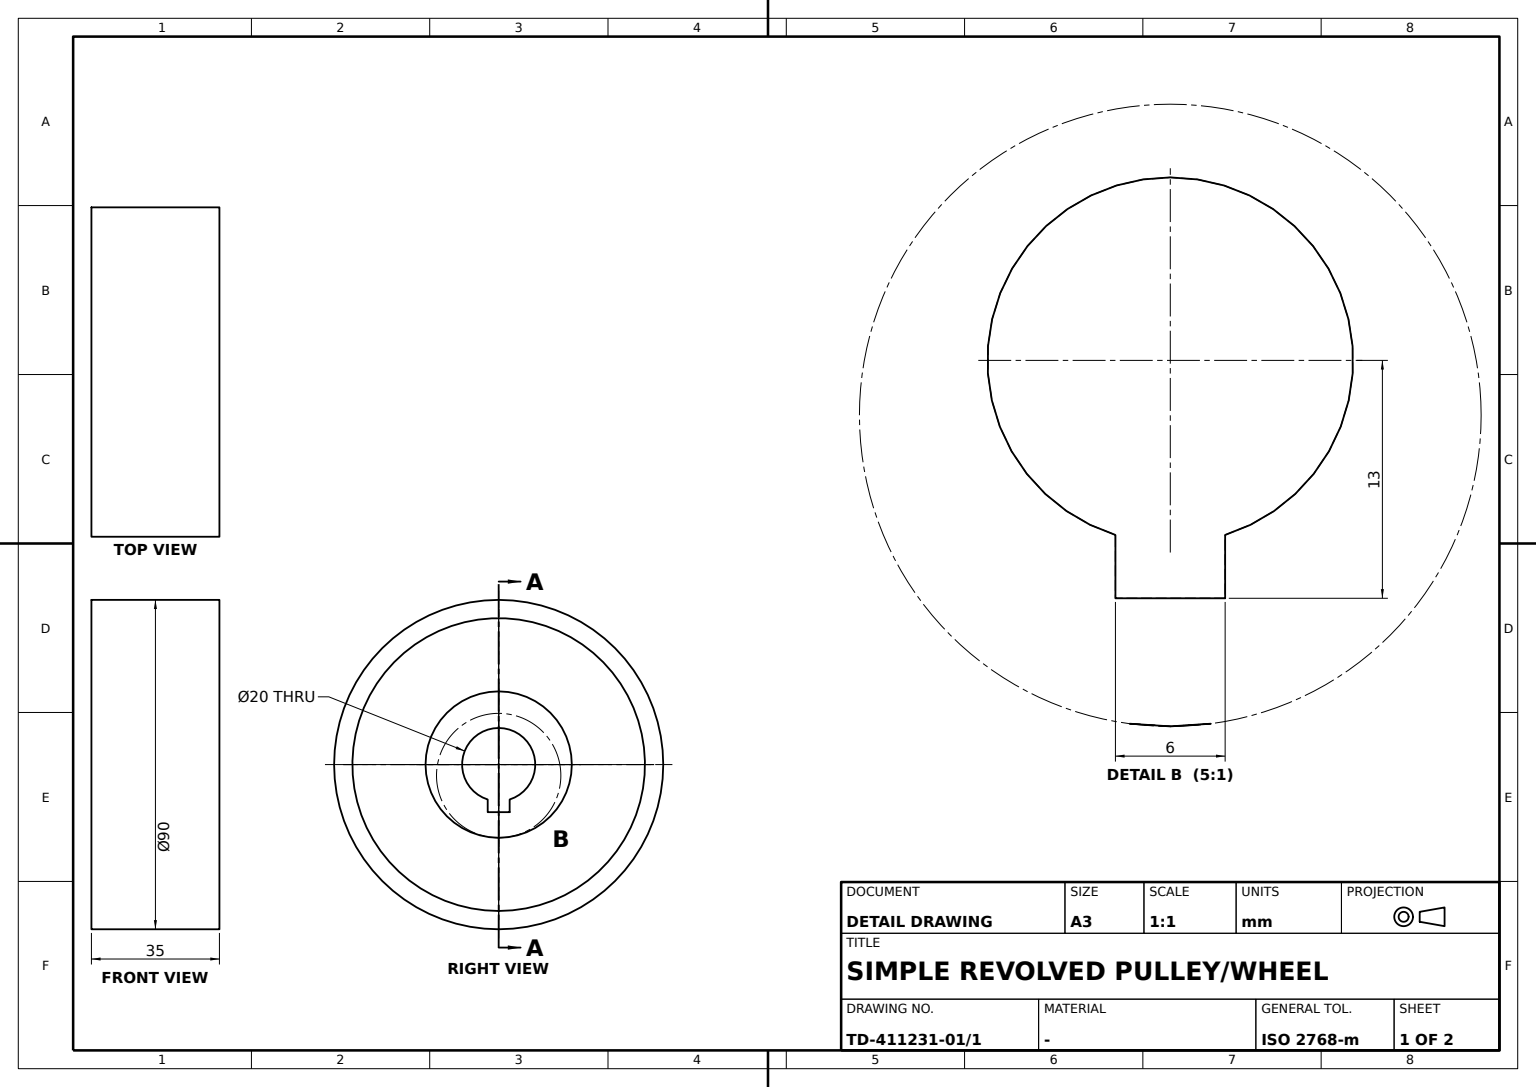
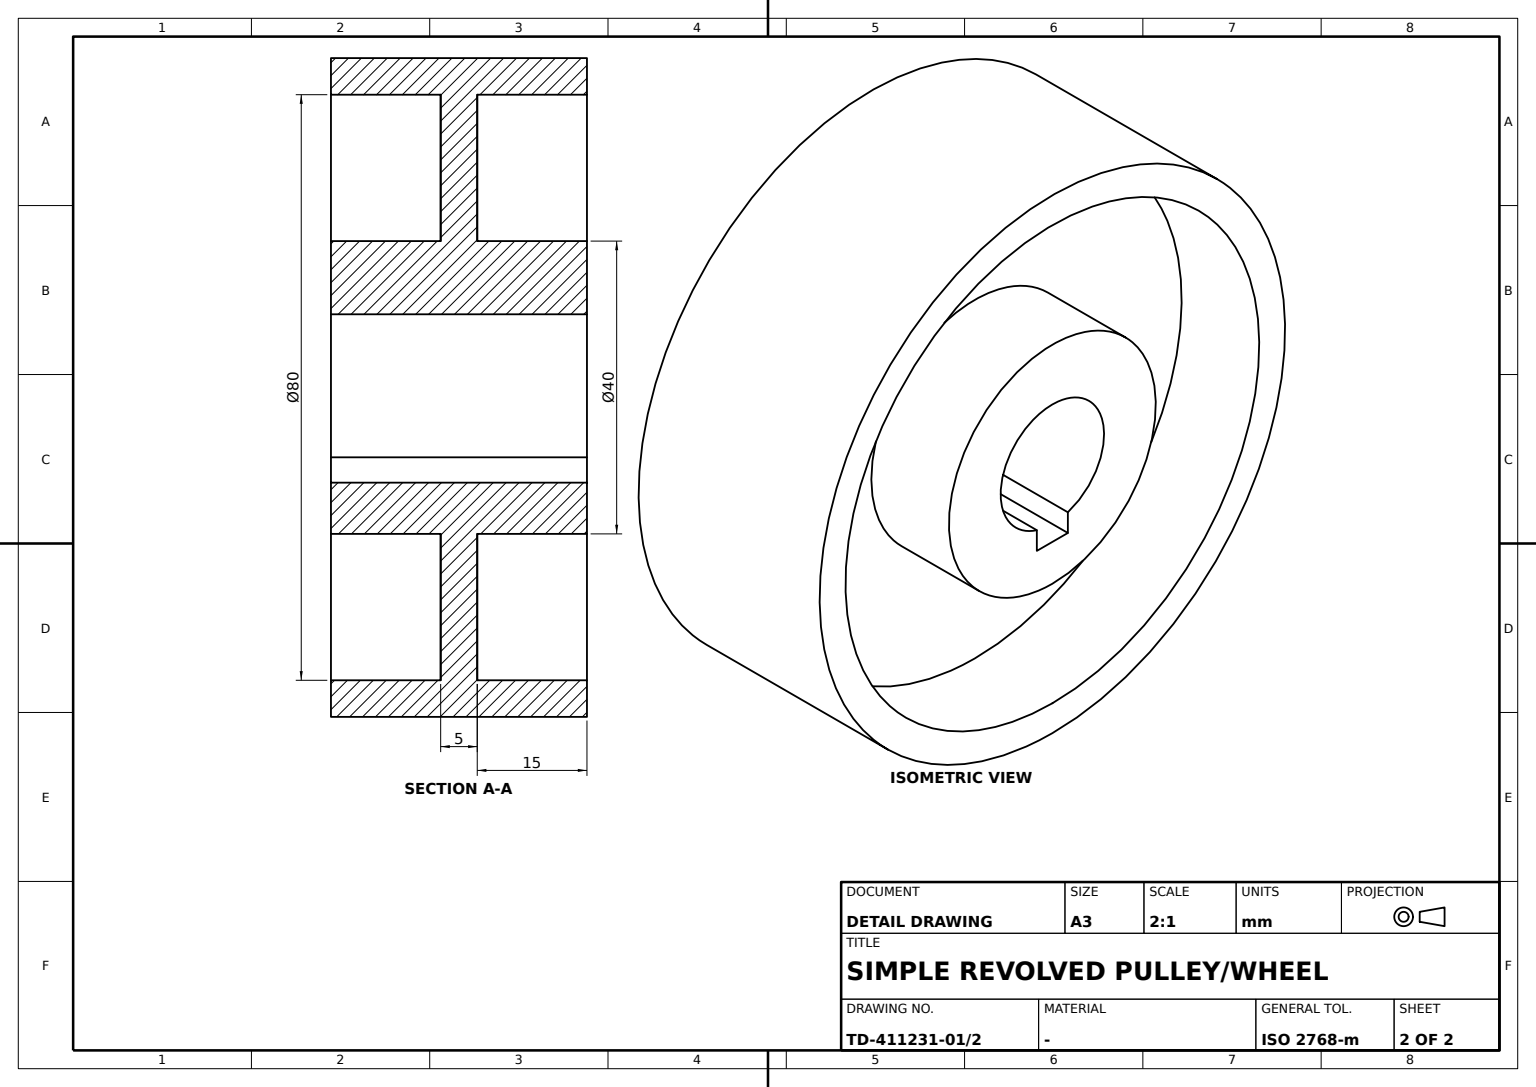
ISO-10303-21;
HEADER;
FILE_DESCRIPTION((''),'2;1');
FILE_NAME('','',(''),(''),'','','');
FILE_SCHEMA(('AUTOMOTIVE_DESIGN'));
ENDSEC;
DATA;
#1=APPLICATION_CONTEXT('');
#2=PRODUCT_CONTEXT('',#1,'mechanical');
#3=PRODUCT('','','',(#2));
#4=PRODUCT_DEFINITION_FORMATION('','',#3);
#5=PRODUCT_DEFINITION_CONTEXT('',#1,'design');
#6=PRODUCT_DEFINITION('','',#4,#5);
#7=PRODUCT_DEFINITION_SHAPE('','',#6);
#8=(LENGTH_UNIT()NAMED_UNIT(*)SI_UNIT(.MILLI.,.METRE.));
#9=(NAMED_UNIT(*)PLANE_ANGLE_UNIT()SI_UNIT($,.RADIAN.));
#10=(NAMED_UNIT(*)SI_UNIT($,.STERADIAN.)SOLID_ANGLE_UNIT());
#11=UNCERTAINTY_MEASURE_WITH_UNIT(LENGTH_MEASURE(0.005),#8,'distance_accuracy_value','');
#12=(GEOMETRIC_REPRESENTATION_CONTEXT(3)GLOBAL_UNCERTAINTY_ASSIGNED_CONTEXT((#11))GLOBAL_UNIT_ASSIGNED_CONTEXT((#8,#9,#10))REPRESENTATION_CONTEXT('',''));
#13=CARTESIAN_POINT('',(17.5,-3.,-13.));
#14=VERTEX_POINT('',#13);
#15=CARTESIAN_POINT('',(-17.5,-3.,-13.));
#16=VERTEX_POINT('',#15);
#17=DIRECTION('',(-1.,0.,0.));
#18=VECTOR('',#17,1000.);
#19=LINE('',#13,#18);
#20=EDGE_CURVE('',#14,#16,#19,.T.);
#21=ORIENTED_EDGE('',*,*,#20,.T.);
#22=CARTESIAN_POINT('',(-17.5,-3.,-9.539392));
#23=VERTEX_POINT('',#22);
#24=CARTESIAN_POINT('',(-17.5,-3.,-6.63467));
#25=DIRECTION('',(0.,0.,-1.));
#26=VECTOR('',#25,1000.);
#27=LINE('',#24,#26);
#28=EDGE_CURVE('',#23,#16,#27,.T.);
#29=ORIENTED_EDGE('',*,*,#28,.F.);
#30=CARTESIAN_POINT('',(17.5,-3.,-9.539392));
#31=VERTEX_POINT('',#30);
#32=DIRECTION('',(1.,0.,0.));
#33=VECTOR('',#32,1000.);
#34=LINE('',#22,#33);
#35=EDGE_CURVE('',#23,#31,#34,.T.);
#36=ORIENTED_EDGE('',*,*,#35,.T.);
#37=CARTESIAN_POINT('',(17.5,-3.,-6.63467));
#38=LINE('',#37,#26);
#39=EDGE_CURVE('',#31,#14,#38,.T.);
#40=ORIENTED_EDGE('',*,*,#39,.T.);
#41=EDGE_LOOP('',(#21,#29,#36,#40));
#42=FACE_BOUND('',#41,.T.);
#43=DIRECTION('',(0.,1.,0.));
#44=AXIS2_PLACEMENT_3D('',#37,#43,#25);
#45=PLANE('',#44);
#46=ADVANCED_FACE('',(#42),#45,.T.);
#47=CARTESIAN_POINT('',(17.5,0.,-45.));
#48=VERTEX_POINT('',#47);
#49=CARTESIAN_POINT('',(17.5,0.,0.));
#50=AXIS2_PLACEMENT_3D('',#49,#32,#25);
#51=CIRCLE('',#50,45.);
#52=EDGE_CURVE('',#48,#48,#51,.T.);
#53=ORIENTED_EDGE('',*,*,#52,.T.);
#54=EDGE_LOOP('',(#53));
#55=FACE_BOUND('',#54,.T.);
#56=CARTESIAN_POINT('',(17.5,0.,-40.));
#57=VERTEX_POINT('',#56);
#58=CIRCLE('',#50,40.);
#59=EDGE_CURVE('',#57,#57,#58,.T.);
#60=ORIENTED_EDGE('',*,*,#59,.F.);
#61=EDGE_LOOP('',(#60));
#62=FACE_BOUND('',#61,.T.);
#63=CARTESIAN_POINT('',(17.5,20.,0.));
#64=AXIS2_PLACEMENT_3D('',#63,#32,#43);
#65=PLANE('',#64);
#66=ADVANCED_FACE('',(#55,#62),#65,.T.);
#67=ORIENTED_EDGE('',*,*,#52,.F.);
#68=EDGE_LOOP('',(#67));
#69=FACE_BOUND('',#68,.T.);
#70=CARTESIAN_POINT('',(-17.5,0.,-45.));
#71=VERTEX_POINT('',#70);
#72=CARTESIAN_POINT('',(-17.5,0.,0.));
#73=AXIS2_PLACEMENT_3D('',#72,#32,#25);
#74=CIRCLE('',#73,45.);
#75=EDGE_CURVE('',#71,#71,#74,.T.);
#76=ORIENTED_EDGE('',*,*,#75,.T.);
#77=EDGE_LOOP('',(#76));
#78=FACE_BOUND('',#77,.T.);
#79=CARTESIAN_POINT('',(0.,0.,0.));
#80=AXIS2_PLACEMENT_3D('',#79,#32,#43);
#81=CYLINDRICAL_SURFACE('',#80,45.);
#82=ADVANCED_FACE('',(#69,#78),#81,.T.);
#83=CARTESIAN_POINT('',(-17.5,0.,-40.));
#84=VERTEX_POINT('',#83);
#85=CIRCLE('',#73,40.);
#86=EDGE_CURVE('',#84,#84,#85,.T.);
#87=ORIENTED_EDGE('',*,*,#86,.F.);
#88=EDGE_LOOP('',(#87));
#89=FACE_BOUND('',#88,.T.);
#90=CARTESIAN_POINT('',(-2.5,0.,-40.));
#91=VERTEX_POINT('',#90);
#92=CARTESIAN_POINT('',(-2.5,0.,0.));
#93=AXIS2_PLACEMENT_3D('',#92,#32,#25);
#94=CIRCLE('',#93,40.);
#95=EDGE_CURVE('',#91,#91,#94,.T.);
#96=ORIENTED_EDGE('',*,*,#95,.T.);
#97=EDGE_LOOP('',(#96));
#98=FACE_BOUND('',#97,.T.);
#99=CYLINDRICAL_SURFACE('',#80,40.);
#100=ADVANCED_FACE('',(#89,#98),#99,.F.);
#101=CARTESIAN_POINT('',(17.5,3.,-13.));
#102=VERTEX_POINT('',#101);
#103=DIRECTION('',(0.,-1.,0.));
#104=VECTOR('',#103,1000.);
#105=LINE('',#101,#104);
#106=EDGE_CURVE('',#102,#14,#105,.T.);
#107=ORIENTED_EDGE('',*,*,#106,.T.);
#108=ORIENTED_EDGE('',*,*,#39,.F.);
#109=CARTESIAN_POINT('',(17.5,3.,-9.539392));
#110=VERTEX_POINT('',#109);
#111=CIRCLE('',#50,10.);
#112=EDGE_CURVE('',#110,#31,#111,.T.);
#113=ORIENTED_EDGE('',*,*,#112,.F.);
#114=DIRECTION('',(0.,0.,1.));
#115=VECTOR('',#114,1000.);
#116=LINE('',#101,#115);
#117=EDGE_CURVE('',#102,#110,#116,.T.);
#118=ORIENTED_EDGE('',*,*,#117,.F.);
#119=EDGE_LOOP('',(#107,#108,#113,#118));
#120=FACE_BOUND('',#119,.T.);
#121=CARTESIAN_POINT('',(17.5,0.,-20.));
#122=VERTEX_POINT('',#121);
#123=CIRCLE('',#50,20.);
#124=EDGE_CURVE('',#122,#122,#123,.T.);
#125=ORIENTED_EDGE('',*,*,#124,.T.);
#126=EDGE_LOOP('',(#125));
#127=FACE_BOUND('',#126,.T.);
#128=ADVANCED_FACE('',(#120,#127),#65,.T.);
#129=ORIENTED_EDGE('',*,*,#112,.T.);
#130=ORIENTED_EDGE('',*,*,#35,.F.);
#131=CARTESIAN_POINT('',(-17.5,3.,-9.539392));
#132=VERTEX_POINT('',#131);
#133=CIRCLE('',#73,10.);
#134=EDGE_CURVE('',#132,#23,#133,.T.);
#135=ORIENTED_EDGE('',*,*,#134,.F.);
#136=LINE('',#109,#33);
#137=EDGE_CURVE('',#110,#132,#136,.F.);
#138=ORIENTED_EDGE('',*,*,#137,.F.);
#139=EDGE_LOOP('',(#129,#130,#135,#138));
#140=FACE_BOUND('',#139,.T.);
#141=CYLINDRICAL_SURFACE('',#80,10.);
#142=ADVANCED_FACE('',(#140),#141,.F.);
#143=CARTESIAN_POINT('',(-17.5,3.,-13.));
#144=VERTEX_POINT('',#143);
#145=LINE('',#143,#104);
#146=EDGE_CURVE('',#144,#16,#145,.T.);
#147=ORIENTED_EDGE('',*,*,#146,.T.);
#148=ORIENTED_EDGE('',*,*,#20,.F.);
#149=ORIENTED_EDGE('',*,*,#106,.F.);
#150=LINE('',#101,#18);
#151=EDGE_CURVE('',#102,#144,#150,.T.);
#152=ORIENTED_EDGE('',*,*,#151,.T.);
#153=EDGE_LOOP('',(#147,#148,#149,#152));
#154=FACE_BOUND('',#153,.T.);
#155=AXIS2_PLACEMENT_3D('',#101,#25,#103);
#156=PLANE('',#155);
#157=ADVANCED_FACE('',(#154),#156,.F.);
#158=CARTESIAN_POINT('',(2.5,0.,-40.));
#159=VERTEX_POINT('',#158);
#160=CARTESIAN_POINT('',(2.5,0.,0.));
#161=AXIS2_PLACEMENT_3D('',#160,#32,#25);
#162=CIRCLE('',#161,40.);
#163=EDGE_CURVE('',#159,#159,#162,.T.);
#164=ORIENTED_EDGE('',*,*,#163,.F.);
#165=EDGE_LOOP('',(#164));
#166=FACE_BOUND('',#165,.T.);
#167=ORIENTED_EDGE('',*,*,#59,.T.);
#168=EDGE_LOOP('',(#167));
#169=FACE_BOUND('',#168,.T.);
#170=ADVANCED_FACE('',(#166,#169),#99,.F.);
#171=ORIENTED_EDGE('',*,*,#124,.F.);
#172=EDGE_LOOP('',(#171));
#173=FACE_BOUND('',#172,.T.);
#174=CARTESIAN_POINT('',(2.5,0.,-20.));
#175=VERTEX_POINT('',#174);
#176=CIRCLE('',#161,20.);
#177=EDGE_CURVE('',#175,#175,#176,.T.);
#178=ORIENTED_EDGE('',*,*,#177,.T.);
#179=EDGE_LOOP('',(#178));
#180=FACE_BOUND('',#179,.T.);
#181=CYLINDRICAL_SURFACE('',#80,20.);
#182=ADVANCED_FACE('',(#173,#180),#181,.T.);
#183=ORIENTED_EDGE('',*,*,#177,.F.);
#184=EDGE_LOOP('',(#183));
#185=FACE_BOUND('',#184,.T.);
#186=ORIENTED_EDGE('',*,*,#163,.T.);
#187=EDGE_LOOP('',(#186));
#188=FACE_BOUND('',#187,.T.);
#189=CARTESIAN_POINT('',(2.5,40.,0.));
#190=AXIS2_PLACEMENT_3D('',#189,#32,#43);
#191=PLANE('',#190);
#192=ADVANCED_FACE('',(#185,#188),#191,.T.);
#193=CARTESIAN_POINT('',(-17.5,0.,-20.));
#194=VERTEX_POINT('',#193);
#195=CIRCLE('',#73,20.);
#196=EDGE_CURVE('',#194,#194,#195,.T.);
#197=ORIENTED_EDGE('',*,*,#196,.F.);
#198=EDGE_LOOP('',(#197));
#199=FACE_BOUND('',#198,.T.);
#200=ORIENTED_EDGE('',*,*,#28,.T.);
#201=ORIENTED_EDGE('',*,*,#146,.F.);
#202=LINE('',#143,#115);
#203=EDGE_CURVE('',#144,#132,#202,.T.);
#204=ORIENTED_EDGE('',*,*,#203,.T.);
#205=ORIENTED_EDGE('',*,*,#134,.T.);
#206=EDGE_LOOP('',(#200,#201,#204,#205));
#207=FACE_BOUND('',#206,.T.);
#208=CARTESIAN_POINT('',(-17.5,45.,0.));
#209=AXIS2_PLACEMENT_3D('',#208,#32,#43);
#210=PLANE('',#209);
#211=ADVANCED_FACE('',(#199,#207),#210,.F.);
#212=CARTESIAN_POINT('',(-2.5,0.,-20.));
#213=VERTEX_POINT('',#212);
#214=CIRCLE('',#93,20.);
#215=EDGE_CURVE('',#213,#213,#214,.T.);
#216=ORIENTED_EDGE('',*,*,#215,.T.);
#217=EDGE_LOOP('',(#216));
#218=FACE_BOUND('',#217,.T.);
#219=ORIENTED_EDGE('',*,*,#95,.F.);
#220=EDGE_LOOP('',(#219));
#221=FACE_BOUND('',#220,.T.);
#222=CARTESIAN_POINT('',(-2.5,40.,0.));
#223=AXIS2_PLACEMENT_3D('',#222,#32,#43);
#224=PLANE('',#223);
#225=ADVANCED_FACE('',(#218,#221),#224,.F.);
#226=ORIENTED_EDGE('',*,*,#196,.T.);
#227=EDGE_LOOP('',(#226));
#228=FACE_BOUND('',#227,.T.);
#229=ORIENTED_EDGE('',*,*,#215,.F.);
#230=EDGE_LOOP('',(#229));
#231=FACE_BOUND('',#230,.T.);
#232=ADVANCED_FACE('',(#228,#231),#181,.T.);
#233=ORIENTED_EDGE('',*,*,#137,.T.);
#234=ORIENTED_EDGE('',*,*,#203,.F.);
#235=ORIENTED_EDGE('',*,*,#151,.F.);
#236=ORIENTED_EDGE('',*,*,#117,.T.);
#237=EDGE_LOOP('',(#233,#234,#235,#236));
#238=FACE_BOUND('',#237,.T.);
#239=AXIS2_PLACEMENT_3D('',#101,#103,#114);
#240=PLANE('',#239);
#241=ADVANCED_FACE('',(#238),#240,.T.);
#242=ORIENTED_EDGE('',*,*,#75,.F.);
#243=EDGE_LOOP('',(#242));
#244=FACE_BOUND('',#243,.T.);
#245=ORIENTED_EDGE('',*,*,#86,.T.);
#246=EDGE_LOOP('',(#245));
#247=FACE_BOUND('',#246,.T.);
#248=ADVANCED_FACE('',(#244,#247),#210,.F.);
#249=CLOSED_SHELL('',(#46,#66,#82,#100,#128,#142,#157,#170,#182,#192,#211,#225,#232,#241,#248));
#250=MANIFOLD_SOLID_BREP('',#249);
#251=ADVANCED_BREP_SHAPE_REPRESENTATION('',(#250),#12);
#252=SHAPE_DEFINITION_REPRESENTATION(#7,#251);
ENDSEC;
END-ISO-10303-21;
